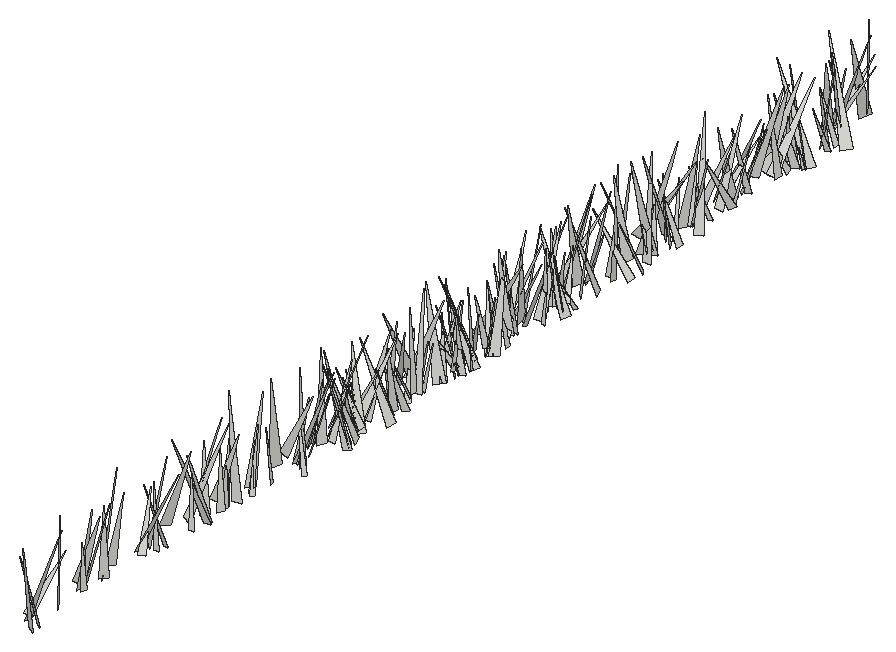
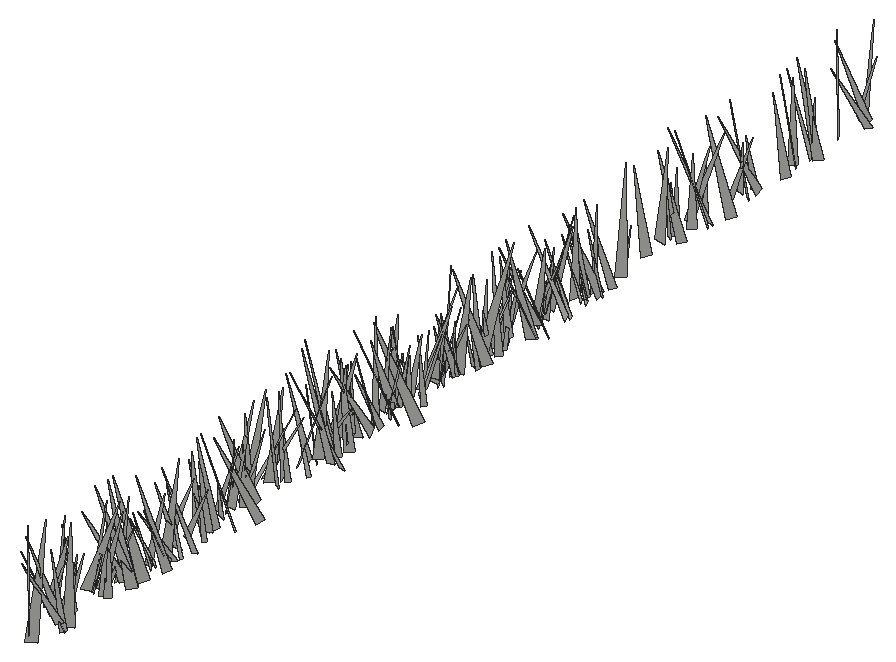
# SketchUp Ruby script. Lengths in inches.
U = 1.inch
M = Sketchup.active_model
def pt(a) = Geom::Point3d.new(a.map { |v| v * U })
def face(e, loops, mat)
  f = e.add_face(loops[0].map { |a| pt(a) })
  loops[1..].each { |l| e.add_face(l.map { |a| pt(a) }).erase! }
  f.material = f.back_material = mat if mat
  f
end
# faces: each face lists its corners as indices into pts; further lists are holes
def faces(e, pts, list, mat = nil) = list.each { |f| face(e, (f[0].is_a?(Array) ? f : [f]).map { |l| l.map { |i| pts[i] } }, mat) }
# xy, xz, yz: faces in a plane at the given z, y or x. An outline is a flat list of corners, or four numbers for a rectangle; further outlines are holes
def ring(l) = l.size == 4 ? [[l[0], l[1]], [l[2], l[1]], [l[2], l[3]], [l[0], l[3]]] : l.each_slice(2).to_a
def flat(e, list, mat, &to3) = list.each { |f| face(e, (f[0].is_a?(Array) ? f : [f]).map { |l| ring(l).map { |u, v| to3.(u, v) } }, mat) }
def xy(e, z, list, mat = nil) = flat(e, list, mat) { |x, y| [x, y, z] }
def xz(e, y, list, mat = nil) = flat(e, list, mat) { |x, z| [x, y, z] }
def yz(e, x, list, mat = nil) = flat(e, list, mat) { |y, z| [x, y, z] }
def lines(e, pts, list) = list.each { |a, b| e.add_line(pt(pts[a]), pt(pts[b])) }
# prism: a flat outline (further loops are holes) pulled along v
def prism(e, loops, v, mat = nil)
  f = face(e, loops, mat); d = Geom::Vector3d.new(v.map { |x| x * U })
  f.pushpull(f.normal.samedirection?(d) ? d.length : -d.length)
end
def box(e, o, s, mat = nil) = prism(e, [[o, [o[0] + s[0], o[1], o[2]], [o[0] + s[0], o[1] + s[1], o[2]], [o[0], o[1] + s[1], o[2]]]], [0, 0, s[2]], mat)
def at(x, y, z, deg = 0) = Geom::Transformation.translation(pt([x, y, z])) * Geom::Transformation.rotation(ORIGIN, Z_AXIS, deg.degrees)
def axes(o, x, y, z) = Geom::Transformation.new([*x, 0, *y, 0, *z, 0, *pt(o).to_a, 1])
def part(name) = M.definitions.add(name)
# library, detail: a bought-in or finely detailed component or shape, given as its bounding box
def library(name, o, s) = part(name).tap { |d| box(d.entities, o, s) }
def detail(e, o, s) = box(e.add_group.entities, o, s)
def put(e, d, t, mat = nil) = e.add_instance(d, t).tap { |i| i.material = mat if mat }
def group(e, t, mat = nil) = e.add_group.tap { |g| g.transformation = t; g.material = mat if mat }.entities
root = M.entities
c1 = part("fur_instance\#9")
p = [[0.8125,0,1.79],[0.67,-0.02,1.48],[0,-0.11,0],[0,0.11,0]]
faces(c1.entities,p,[[0,1,2,3]])
put(root,c1,axes([157.47,112.2,-27.1],[-4.17455,0.44699,1.70239],[0.80041,4.38471,0.81146],[1.56757,-1.04848,4.11925]))
put(root,c1,axes([157.79,64.41,-28.22],[-3.70453,-1.18645,1.17686],[-1.32576,3.8289,-0.31316],[1.01735,0.66938,3.87726]))
put(root,c1,axes([155.74,183.69,-28.22],[3.44417,-6.15496,0.43731],[-6.17002,-3.42915,0.33004],[0.07525,0.54268,7.04535]))
put(root,c1,axes([158.09,92.44,-28.22],[-4.08982,2.78235,0.32679],[2.66533,4.04258,-1.06229],[0.86271,0.7007,4.83111]))
put(root,c1,axes([156.51,123.77,-27.1],[4.13906,-0.88394,1.08396],[-0.87234,-4.27812,-0.15771],[-1.09332,0.06702,4.22946]))
put(root,c1,axes([155.58,185.05,-28.22],[5.53978,-0.90724,0.62547],[-0.85463,-5.56113,-0.49688],[-0.69563,-0.39269,5.59154]))
put(root,c1,axes([157.55,75.13,-27.1],[6.19428,-1.57461,3.33029],[-1.87234,-6.95675,0.19327],[-3.17247,1.03131,6.38836]))
put(root,c1,axes([157.63,117.22,-27.1],[3.93388,5.26717,1.14139],[4.90502,-4.08461,1.94372],[-2.23307,0.30691,6.28017]))
put(root,c1,axes([153.48,151.58,-27.1],[5.8756,3.65861,0.2575],[3.32747,-5.11292,-3.2803],[1.54262,-2.90637,6.0949]))
put(root,c1,axes([159.0625,112.28,-28.22],[-5.62081,-1.07857,0.79033],[-1.22962,5.511,-1.22409],[0.52534,1.35906,5.59093]))
put(root,c1,axes([155.79,118.01,-27.1],[4.34496,-0.35551,0.43941],[-0.4633,-4.19131,1.19014],[-0.32376,1.22666,4.19388]))
put(root,c1,axes([155.21,79.86,-27.1],[6.72288,3.05704,0.61475],[3.02645,-6.7488,0.46346],[-0.75102,0.16938,7.37074]))
put(root,c1,axes([157.85,82.52,-28.22],[-2.17091,-2.72609,1.07786],[-2.90812,2.17161,-0.36485],[0.36901,1.07644,3.46573]))
put(root,c1,axes([157.48,28.99,-27.1],[5.31201,5.41879,2.20999],[5.24419,-5.73235,1.45032],[-2.59727,-0.49162,7.44831]))
put(root,c1,axes([157.34,50.82,-27.1],[2.70237,-4.42657,2.31196],[-4.83243,-2.98105,-0.05917],[-1.25989,1.93941,5.18593]))
put(root,c1,axes([156.33,124.09,-28.22],[3.53738,-5.32848,1.99163],[-5.66565,-3.51029,0.67133],[-0.50966,2.039,6.36044]))
put(root,c1,axes([158.61,155.47,-28.22],[-0.5806,-4.0301,0.94816],[-3.96701,0.26756,-1.29192],[-1.18471,1.07913,3.86131]))
put(root,c1,axes([156.16,32.51,-27.1],[5.31281,-2.73186,1.51927],[-2.91837,-5.40827,0.48055],[-1.11999,1.13346,5.95467]))
put(root,c1,axes([159.02,142.16,-27.1],[-5.68888,-0.08485,0.69236],[-0.12916,5.71868,-0.36046],[0.68548,0.37338,5.67808]))
put(root,c1,axes([158.48,82.14,-28.22],[-4.49758,4.50366,1.60112],[4.72062,4.53017,0.51777],[0.74986,-1.50644,6.34374]))
put(root,c1,axes([158.22,98.96,-28.22],[-5.45216,4.70878,2.71596],[5.23215,5.58914,0.81316],[1.47433,-2.42158,7.15803]))
put(root,c1,axes([158.49,56.12,-27.1],[-0.94907,-6.99906,3.73248],[-7.88487,0.42284,-1.21201],[-0.8643,3.82797,6.95835]))
put(root,c1,axes([153.68,146.02,-28.22],[4.55,-4.60588,0.41001],[-4.16176,-3.82822,3.1795],[2.01545,2.49305,5.6398]))
put(root,c1,axes([157.15,95.66,-27.1],[4.52461,-6.7861,0.00105],[-6.53347,-4.35651,-2.20405],[-1.83437,-1.22185,7.85273]))
put(root,c1,axes([156.55,70.85,-28.22],[2.00613,4.44684,1.43472],[4.67253,-1.91449,-0.59961],[-0.01581,-1.5549,4.84142]))
put(root,c1,axes([154.18,128.22,-28.22],[3.82071,6.83533,0.31448],[6.59967,-3.58608,-2.23672],[1.80694,-1.35528,7.50444]))
put(root,c1,axes([154.97,83.86,-28.22],[3.75203,3.55416,0.24846],[3.4305,-3.50645,-1.64561],[0.96201,-1.35805,4.89916]))
put(root,c1,axes([155.06,129.59,-27.1],[-0.81294,-7.33898,4.00432],[-7.82592,2.08335,2.22952],[2.94113,3.51498,7.03923]))
put(root,c1,axes([158.54,148.17,-28.22],[0.48963,4.22721,0.04806],[3.94805,-0.47454,1.51627],[-1.51146,0.12987,3.97618]))
put(root,c1,axes([159.07,49.21,-27.1],[-1.75901,-6.72397,0.92553],[-6.70142,1.56883,-1.33876],[-1.07676,1.22044,6.82009]))
put(root,c1,axes([156.52,66.78,-27.1],[6.94101,-3.43299,1.84422],[-3.2352,-7.17632,-1.18245],[-2.17258,-0.28153,7.65277]))
put(root,c1,axes([157.6,37.26,-27.1],[-2.09366,4.25191,0.8072],[4.26644,2.17826,-0.40798],[0.72654,-0.53866,4.72184]))
put(root,c1,axes([155.98,161.09,-28.22],[-0.54715,4.89077,0.10405],[4.53126,0.54616,-1.84371],[1.84341,0.10915,4.56287]))
put(root,c1,axes([158.66,108.89,-28.22],[-1.86757,4.60063,0.33127],[4.58089,1.80817,0.71369],[-0.53944,-0.57279,4.91369]))
put(root,c1,axes([158.64,41.03,-27.1],[-2.25031,-4.2676,0.76277],[-4.32128,2.13921,-0.77999],[-0.34742,1.03417,4.76108]))
put(root,c1,axes([158.95,81.81,-27.1],[-4.51725,1.3418,0.80765],[1.52463,4.33149,1.33117],[0.35811,-1.51528,4.52039]))
put(root,c1,axes([158.38,39.37,-27.1],[0.93593,4.40998,1.37185],[4.37962,-1.29175,1.16453],[-1.46587,-1.0437,4.3552]))
put(root,c1,axes([157.36,152.39,-28.22],[-2.00411,5.21831,1.67163],[5.38658,2.20263,-0.41796],[1.00489,-1.39973,5.57427]))
put(root,c1,axes([153.78,112.64,-28.22],[6.07863,-4.42165,0.21276],[-4.21796,-5.67554,2.55792],[1.3435,2.18706,7.06807]))
put(root,c1,axes([156.63,138.79,-27.1],[-3.30417,-4.76212,3.2823],[-5.25525,4.05058,0.5865],[2.41528,2.29867,5.7664]))
put(root,c1,axes([158.08,70.5625,-28.22],[-6.67663,-0.80436,2.4344],[-1.05353,7.05179,-0.55944],[2.33738,0.88086,6.7016]))
put(root,c1,axes([158.02,164.22,-28.22],[0.08099,-5.17118,1.20761],[-5.27072,-0.22549,-0.61212],[-0.64729,1.18913,5.13546]))
put(root,c1,axes([160.05,174.42,-28.22],[-5.06971,5.94983,1.91077],[6.22333,4.58369,2.23904],[-0.56711,-2.88838,7.48926]))
put(root,c1,axes([156.17,154.67,-28.22],[0.84418,-3.62493,0.18375],[-3.45271,-0.74384,1.18829],[1.11924,0.43944,3.52714]))
put(root,c1,axes([155.01,45.44,-27.1],[6.03076,-3.95506,0.64167],[-4.00583,-5.92637,1.12057],[0.08689,1.28836,7.12438]))
put(root,c1,axes([157.19,118.1875,-28.22],[6.83312,3.40706,1.30672],[2.45514,-6.34476,3.70451],[-2.69961,2.8536,6.67654]))
put(root,c1,axes([155.23,157.86,-28.22],[2.52048,5.79703,1.2985],[5.75928,-2.03853,-2.07834],[1.45681,-1.97061,5.96983]))
put(root,c1,axes([155.59,160.3,-28.22],[4.89387,1.35478,0.49174],[1.44124,-4.60961,-1.64362],[-0.00784,-1.71558,4.80457]))
put(root,c1,axes([158.59,92.4,-27.1],[-3.47143,-2.84551,0.09651],[-2.81271,3.45107,0.57956],[0.4415,-0.38766,4.45106]))
put(root,c1,axes([156.99,161.96,-28.22],[3.26606,-6.16963,0.62937],[-6.14796,-3.31446,-0.58694],[-0.81426,0.27855,6.95607]))
put(root,c1,axes([158.59,106.58,-28.22],[-5.73536,-5.62008,0.65862],[-5.46135,5.74328,1.44982],[1.48081,-0.58562,7.89796]))
put(root,c1,axes([158.91,13.99,-27.1],[-3.27995,-3.84872,1.10692],[-4.00472,3.15616,-0.89264],[0.01123,1.42196,4.97734]))
put(root,c1,axes([158.91,183.92,-27.1],[-3.27995,-3.84872,1.10692],[-4.00472,3.15616,-0.89264],[0.01123,1.42196,4.97734]))
put(root,c1,axes([156.54,126.08,-28.22],[4.24921,-1.39082,0.67887],[-1.35455,-4.30166,-0.33452],[-0.74864,-0.11098,4.4585]))
put(root,c1,axes([158.44,93.38,-27.1],[-5.81537,-0.03657,1.70774],[-0.23888,6.01751,-0.6846],[1.69135,0.72416,5.77505]))
put(root,c1,axes([158.31,102.99,-28.22],[-4.48519,-3.52054,0.94744],[-3.42145,4.58335,0.83384],[1.25916,-0.08621,5.64055]))
put(root,c1,axes([156.49,75.13,-27.1],[4.35259,2.65064,0.87547],[2.69973,-4.40951,-0.0717],[-0.70982,-0.51745,5.09567]))
put(root,c1,axes([158.14,54.52,-27.1],[1.43677,3.63281,1.03111],[3.57622,-1.66329,0.8769],[-1.21291,-0.60083,3.80693]))
put(root,c1,axes([157.74,180.98,-28.22],[-1.67476,-3.89018,1.26522],[-4.03938,1.78862,0.15259],[0.64624,1.09838,4.23261]))
put(root,c1,axes([157.96,100.26,-27.1],[1.56672,2.93333,1.48069],[3.11219,-1.85095,0.37383],[-1.05412,-1.105,3.30444]))
put(root,c1,axes([156.88,100.88,-27.1],[4.55494,-1.38322,1.77977],[-1.90749,-4.50337,1.38185],[-1.20098,1.9065,4.55536]))
put(root,c1,axes([158.19,112.65,-27.1],[-3.4412,6.39637,0.09759],[6.32165,3.41718,-1.06042],[0.97968,0.41743,7.18546]))
put(root,c1,axes([158.67,173.29,-28.22],[0.96308,-5.75121,1.64983],[-5.7805,-1.32563,-1.24675],[-1.54408,1.37555,5.69645]))
put(root,c1,axes([156.55,73.67,-27.1],[4.95919,2.18923,1.00137],[2.21006,-5.04934,0.09393],[-0.95452,-0.31696,5.4201]))
put(root,c1,axes([154.92,164.02,-28.22],[6.75875,-1.16964,0.00047],[-1.16859,-6.75255,0.29358],[0.0496,0.28936,6.85293]))
put(root,c1,axes([157.71,158.37,-28.22],[0.77683,6.56918,0.32302],[6.56801,-0.79193,0.30978],[-0.34589,-0.28401,6.60769]))
put(root,c1,axes([156.57,84.83,-28.22],[3.10305,4.72146,0.30771],[4.72969,-3.10544,-0.04628],[-0.13026,-0.28259,5.64969]))
put(root,c1,axes([157.29,164.5625,-28.22],[3.89268,2.82638,0.90518],[2.67493,-3.98806,0.94914],[-1.28551,0.26015,4.71599]))
put(root,c1,axes([158.48,102.09,-27.1],[2.70067,-3.13661,0.88183],[-2.51329,-2.73437,-2.02883],[-2.07348,-0.77102,3.60774]))
put(root,c1,axes([156.36,48.83,-27.1],[5.62974,5.25868,1.12192],[5.27805,-5.71471,0.30107],[-1.02693,-0.54292,7.69786]))
put(root,c1,axes([158.54,99.46,-28.22],[-4.5869,1.43943,1.05541],[1.33614,4.69877,-0.60151],[1.18347,0.27406,4.76967]))
put(root,c1,axes([157.04,81.8125,-27.1],[-0.66532,-4.77379,0.4836],[-4.67341,0.75535,1.0268],[1.0873,0.32553,4.70929]))
put(root,c1,axes([160.52,138.84,-28.22],[-5.4011,-4.4458,0.12135],[-4.40164,5.31613,-1.14717],[-0.63674,0.96192,6.9008]))
put(root,c1,axes([158.79,134.85,-28.22],[-7.37531,-1.40171,2.74866],[-2.16749,7.42249,-2.03071],[2.19589,2.61858,7.22747]))
put(root,c1,axes([159.3125,131.0625,-28.22],[-6.20771,-3.16783,0.82777],[-3.08728,6.25411,0.78157],[1.09042,-0.32718,6.92531]))
put(root,c1,axes([156.02,15.29,-27.1],[-0.77489,5.32124,0.74593],[4.8544,1.01638,-2.20776],[2.30365,-0.35187,4.90325]))
put(root,c1,axes([156.02,185.21,-27.1],[-0.77489,5.32124,0.74593],[4.8544,1.01638,-2.20776],[2.30365,-0.35187,4.90325]))
put(root,c1,axes([156.64,174.39,-28.22],[3.91329,-2.80057,0.16354],[-2.76188,-3.89534,-0.61821],[-0.49189,-0.40864,4.7723]))
put(root,c1,axes([156.87,25.13,-27.1],[6.13024,0.22864,1.74835],[0.20896,-6.37456,0.10097],[-1.75081,0.03976,6.13367]))
put(root,c1,axes([157.33,60.35,-27.1],[-5.57842,3.33095,2.99608],[3.28064,6.29556,-0.89096],[3.05108,-0.67911,6.43585]))
put(root,c1,axes([157.11,129.6,-27.1],[6.05759,-4.04132,1.47541],[-3.82561,-6.22554,-1.34569],[-1.96821,-0.33746,7.15653]))
put(root,c1,axes([158.96,80.94,-28.22],[2.56501,3.25674,2.5986],[3.3721,-3.41499,0.95138],[-2.44704,-1.29222,4.03491]))
put(root,c1,axes([159.47,104.85,-28.22],[-5.95975,2.47486,1.75961],[2.91321,5.75356,1.77469],[0.85695,-2.34763,6.20435]))
put(root,c1,axes([156.4375,74.08,-27.1],[5.73568,-0.06882,1.05766],[0.01363,-5.81521,-0.45231],[-1.05981,-0.44725,5.71823]))
put(root,c1,axes([157.63,25.0625,-27.1],[3.35457,-1.66316,1.27005],[-1.64462,-3.57909,-0.343],[-1.29397,0.23728,3.72849]))
put(root,c1,axes([157.97,53.91,-27.1],[-2.87037,3.7349,1.34525],[3.80013,3.06525,-0.40189],[1.14815,-0.80807,4.69329]))
put(root,c1,axes([157.9,144.2,-28.22],[-2.69115,3.5868,1.84623],[3.86426,2.92918,-0.05799],[1.15809,-1.43902,4.48375]))
put(root,c1,axes([157.51,174.43,-28.22],[1.04102,-4.92803,1.21287],[-5.07408,-1.03535,0.14838],[-0.10125,1.21771,5.0346]))
put(root,c1,axes([158.19,138.52,-27.1],[-6.01027,1.97565,2.91231],[2.62602,6.35479,1.10849],[2.3428,-2.05464,6.22879]))
put(root,c1,axes([159.04,181.29,-28.22],[-4.29082,0.07848,0.62907],[0.12494,4.3243,0.31276],[0.62151,-0.32753,4.28013]))
put(root,c1,axes([156.87,96.3,-28.22],[4.1341,0.32333,0.78637],[0.3951,-4.18703,-0.35553],[-0.75288,-0.42186,4.13146]))
put(root,c1,axes([156.06,77.87,-28.22],[4.46845,1.48023,0.19389],[1.49287,-4.43008,-0.58427],[0.00126,-0.6156,4.67084]))
put(root,c1,axes([157.32,163.58,-28.22],[3.29969,3.36632,0.10349],[3.25213,-3.22241,1.12716],[-0.87548,0.71745,4.57707]))
put(root,c1,axes([158.87,93.67,-27.1],[0.5538,7.06628,1.29605],[7.05626,-0.7792,1.23321],[-1.34954,-1.17443,6.97985]))
put(root,c1,axes([156.96,151.4375,-28.22],[6.61649,-1.70465,2.3436],[-2.13195,-6.81989,1.0584],[-1.96294,1.66119,6.75008]))
put(root,c1,axes([158.46,123.48,-27.1],[-4.8782,2.33838,1.88669],[2.5546,5.12175,0.25721],[1.58166,-1.06025,5.40358]))
put(root,c1,axes([157.9,147.11,-27.1],[-0.40558,-7.48594,0.6627],[-7.51279,0.42075,0.15485],[0.19107,0.65318,7.49532]))
put(root,c1,axes([155.63,168.05,-28.22],[6.10397,-4.61293,1.81963],[-4.95361,-5.80478,1.9013],[-0.22786,2.62185,7.41098]))
put(root,c1,axes([159.83,77.6875,-28.22],[-0.65544,-6.57541,2.82853],[-6.91722,-0.14862,-1.94837],[-1.84083,2.89967,6.31422]))
put(root,c1,axes([158.56,172.01,-28.22],[-4.22388,-0.55824,1.0602],[-0.01996,3.91714,1.98304],[1.19803,-1.90295,3.77099]))
put(root,c1,axes([160.77,181.35,-28.22],[-3.56857,7.17935,0.49748],[7.02506,3.35468,1.97986],[-1.56176,-1.31463,7.76903]))
put(root,c1,axes([158.45,169.9,-28.22],[5.59524,-0.57904,3.08549],[-0.36766,-6.38318,-0.53118],[-3.11775,-0.28642,5.59999]))
put(root,c1,axes([159.71,125.71,-28.22],[-0.53868,-3.7535,0.51973],[-3.36849,0.23389,-1.80211],[-1.73555,0.71104,3.33637]))
put(root,c1,axes([155.44,96.09,-27.1],[4.70932,-5.02611,1.74089],[-5.27526,-4.11549,2.38842],[0.68127,2.87596,6.46026]))
put(root,c1,axes([157.375,90.03,-28.22],[4.05773,-0.76512,0.97615],[-0.40955,-3.97873,-1.41614],[-1.1707,-1.26007,3.87881]))
put(root,c1,axes([156.31,108.39,-28.22],[4.66467,-0.77947,0.02704],[-0.7406,-4.47818,-1.32848],[-0.24456,-1.30606,4.53893]))
put(root,c1,axes([157.875,111.09,-27.1],[3.73887,4.62596,1.90486],[4.75099,-4.02818,0.45718],[-1.5672,-1.17533,5.9304]))
put(root,c1,axes([155.71,170.51,-28.22],[4.37755,-6.1842,1.75356],[-6.40379,-4.01166,1.83857],[0.55746,2.47882,7.3503]))
put(root,c1,axes([156.91,101.11,-27.1],[-0.57371,3.97778,1.97621],[4.19128,1.14438,-1.08668],[1.47014,-1.71025,3.86924]))
put(root,c1,axes([157.14,142.68,-28.22],[7.73551,0.03019,2.73159],[-1.01366,-7.58581,2.95441],[-2.53672,3.12332,7.14916]))
put(root,c1,axes([158.25,108.75,-27.1],[1.30026,-4.12004,1.09762],[-4.18224,-1.45572,-0.50983],[-0.82967,0.8811,4.29016]))
put(root,c1,axes([156.68,39.93,-27.1],[-3.91032,-4.73518,3.93684],[-5.20514,5.03349,0.88414],[3.29046,2.33522,6.07707]))
put(root,c1,axes([159.94,151.28,-28.22],[0.30584,8.28043,0.48557],[7.987,-0.4251,2.21855],[-2.2381,-0.38549,7.98355]))
put(root,c1,axes([156.11,169.82,-28.22],[-0.17327,7.80384,1.95788],[7.72096,0.71202,-2.15474],[2.26272,-1.83203,7.50246]))
put(root,c1,axes([159.12,102.66,-28.22],[0.3865,-5.10308,2.42648],[-5.49086,-0.91339,-1.04632],[-1.33405,2.28099,5.00959]))
put(root,c1,axes([159.33,104.625,-28.22],[-5.30333,-1.20318,1.41609],[-1.56427,5.2022,-1.4382],[1.00301,1.75149,5.24448]))
put(root,c1,axes([160.55,136.46,-28.22],[-5.67147,0.82087,0.04901],[0.80443,5.46726,1.5178],[-0.17066,-1.50898,5.5259]))
put(root,c1,axes([156.76,73.66,-28.22],[4.65489,2.00226,0.76997],[2.06003,-4.68544,-0.26978],[-0.59848,-0.55448,5.06006]))
put(root,c1,axes([157.6875,88.79,-27.1],[5.90361,-0.69248,2.28384],[-0.937,-6.27702,0.51884],[-2.19488,0.81708,5.9214]))
put(root,c1,axes([158.9,49.66,-27.1],[-0.82643,-5.48525,0.94931],[-5.54864,0.73423,-0.58792],[-0.44918,1.02229,5.51591]))
put(root,c1,axes([155.74,93.35,-27.1],[6.93671,-0.62868,0.23505],[-0.51232,-6.5363,-2.3628],[-0.4336,-2.33453,6.55213]))
put(root,c1,axes([159.5,174.07,-28.22],[-4.59653,-5.39297,2.39685],[-5.86856,4.49796,-1.13384],[0.62378,2.57709,6.99476]))
put(root,c1,axes([158.375,143.41,-28.22],[1.61042,-7.88282,1.5376],[-7.97737,-1.75156,-0.62458],[-0.92985,1.37466,8.02136]))
put(root,c1,axes([158.36,113.35,-27.1],[-2.64442,5.36733,3.49605],[6.32318,2.79183,0.49668],[1.02376,-3.3795,5.96276]))
put(root,c1,axes([155.4,69.84,-27.1],[1.83372,-5.8574,1.52699],[-5.60076,-1.03656,2.74963],[2.29617,2.14936,5.48737]))
put(root,c1,axes([158.94,119.91,-28.22],[1.77865,4.09096,1.0407],[3.89915,-2.02489,1.29578],[-1.61729,-0.38272,4.26855]))
put(root,c1,axes([158.72,101.15,-27.1],[-4.5247,0.14497,1.56827],[-0.47946,4.4174,-1.79167],[1.5002,1.84904,4.15738]))
put(root,c1,axes([156.78,14.41,-27.1],[6.71372,1.26121,1.18447],[0.98901,-6.69183,1.51954],[-1.41968,1.3025,6.66001]))
put(root,c1,axes([156.78,184.34,-27.1],[6.71372,1.26121,1.18447],[0.98901,-6.69183,1.51954],[-1.41968,1.3025,6.66001]))
put(root,c1,axes([159.57,173.79,-28.22],[-3.7674,-0.4134,0.34529],[-0.49063,3.64055,-0.99453],[0.22227,1.02903,3.6572]))
put(root,c1,axes([157.58,29.26,-27.1],[-3.8078,3.44308,3.43375],[4.19662,4.52997,0.11149],[2.45637,-2.40193,5.13242]))
put(root,c1,axes([159.28,141.24,-28.22],[1.24745,7.40868,1.63783],[7.39275,-1.56046,1.42803],[-1.70827,-1.34297,7.376]))
put(root,c1,axes([157.89,96.03,-28.22],[1.71748,3.11444,0.84575],[3.20742,-1.75327,-0.057],[-0.35706,-0.7688,3.55615]))
put(root,c1,axes([156.57,85.46,-28.22],[3.44666,-5.98968,2.82803],[-6.61551,-2.95389,1.80641],[0.33028,3.33943,6.67028]))
put(root,c1,axes([157.71,113.75,-28.22],[-1.72893,-3.46771,1.76985],[-3.62718,2.13831,0.64633],[1.41454,1.24466,3.82053]))
put(root,c1,axes([158.9,159.82,-28.22],[2.87484,-4.36178,0.57915],[-3.91954,-2.85297,-2.03053],[-1.99945,-0.67874,4.81319]))
put(root,c1,axes([158.51,146.05,-27.1],[-3.07714,-3.38347,1.94932],[-3.73457,3.27489,-0.21099],[1.14047,1.59489,4.5686]))
put(root,c1,axes([157.63,135.36,-28.22],[0.94774,-3.5048,1.15841],[-3.67796,-0.79512,0.60341],[0.31324,1.26803,3.58018]))
put(root,c1,axes([159.375,80.19,-28.22],[-5.8236,-1.97497,1.08531],[-1.72724,5.8434,1.36532],[1.44743,-0.9731,5.99589]))
put(root,c1,axes([157.15,189.85,-28.22],[6.81384,-4.6319,0.82302],[-4.34734,-6.75311,-2.01405],[-1.7979,-1.22528,7.98915]))
put(root,c1,axes([156.03,54.54,-27.1],[3.29636,-5.4576,1.30622],[-5.51274,-2.86598,1.93739],[1.04942,2.08768,6.07437]))
put(root,c1,axes([156.74,70.84,-28.22],[6.92746,0.46404,1.30725],[0.06508,-6.75935,2.05449],[-1.38564,2.00246,6.63205]))
put(root,c1,axes([157.5,19.875,-27.1],[6.08028,3.66314,2.96745],[4.34842,-6.22849,-1.22118],[-1.82087,-2.64225,6.99265]))
put(root,c1,axes([157.5,189.81,-27.1],[6.08028,3.66314,2.96745],[4.34842,-6.22849,-1.22118],[-1.82087,-2.64225,6.99265]))
put(root,c1,axes([158.2,76.42,-27.1],[1.54833,5.59255,0.52827],[5.59137,-1.58705,0.41342],[-0.54067,-0.39706,5.78818]))
put(root,c1,axes([158.46,160.5,-28.22],[2.63197,4.07891,0.20518],[3.86496,-2.5665,1.44292],[-1.31973,0.61842,4.63495]))
put(root,c1,axes([158.1875,108.875,-28.22],[3.3556,2.16226,1.21696],[2.08771,-3.56664,0.58052],[-1.34083,-0.14202,3.94948]))
put(root,c1,axes([158.39,52.87,-27.1],[-3.98978,2.11987,2.03955],[2.3526,4.36264,0.06771],[1.76604,-1.02247,4.51748]))
put(root,c1,axes([156.22,114.16,-28.22],[4.64022,6.0526,0.40907],[6.0581,-4.59639,-0.71102],[0.31728,-0.75645,7.59342]))
put(root,c1,axes([160.21,86.36,-28.22],[-6.51837,1.52305,1.37348],[1.82295,6.39951,1.5551],[0.93967,-1.84981,6.5108]))
put(root,c1,axes([157.97,121.47,-27.1],[0.13174,-4.85064,1.64659],[-5.10405,0.01535,0.4536],[0.43432,1.65178,4.83118]))
put(root,c1,axes([159.04,58.67,-27.1],[-3.45785,1.40655,0.59459],[1.25916,3.45892,-0.85969],[0.86397,0.58836,3.63264]))
put(root,c1,axes([158.06,128.78,-28.22],[3.88828,4.27161,1.82836],[4.44707,-4.1121,0.14976],[-1.3465,-1.2459,5.77433]))
put(root,c1,axes([155.875,26.125,-27.1],[2.64878,-6.42579,1.07864],[-6.29914,-2.22772,2.19734],[1.66585,1.79353,6.59382]))
put(root,c1,axes([156.875,26.32,-27.1],[6.30339,2.19635,1.13005],[2.22882,-6.39265,-0.00763],[-1.06457,-0.37914,6.67507]))
put(root,c1,axes([156.08,127.84,-27.1],[7.78659,2.72532,1.24866],[2.87625,-7.77148,-0.97412],[-0.84485,-1.33952,8.19204]))
put(root,c1,axes([158.98,146.59,-28.22],[-3.81411,-2.18756,1.38745],[-2.30966,3.98998,-0.05835],[1.17299,0.74331,4.39652]))
put(root,c1,axes([156.39,48.22,-27.1],[3.64323,6.95762,0.66244],[6.95502,-3.53547,-1.11744],[0.68929,-1.10109,7.77386]))
put(root,c1,axes([158.66,46.38,-27.1],[-0.06677,3.94377,1.582],[4.24655,0.00562,0.16522],[-0.15123,-1.5834,3.94087]))
put(root,c1,axes([156.25,132.58,-28.22],[5.4983,0.81734,0.21266],[0.84397,-5.26527,-1.58403],[0.03145,-1.59793,5.32824]))
put(root,c1,axes([157.91,120.34,-28.22],[-1.91497,6.86191,1.78883],[6.91485,2.21764,-1.10438],[1.57179,-1.39609,7.03799]))
put(root,c1,axes([159.18,109.38,-28.22],[-5.92088,3.75972,1.43779],[3.50525,6.07307,-1.44586],[1.97886,0.49178,6.86307]))
put(root,c1,axes([160.08,123.2,-28.22],[-6.07802,2.92755,1.98205],[3.37511,5.97833,1.51972],[1.05246,-2.26504,6.57292]))
put(root,c1,axes([158.625,114.35,-27.1],[-1.20745,-5.31811,1.49773],[-5.50418,1.29079,0.14593],[0.47907,1.42653,5.45151]))
put(root,c1,axes([158.65,58.95,-27.1],[0.70725,4.81258,1.31899],[4.97344,-0.78845,0.21001],[-0.40688,-1.27212,4.85974]))
put(root,c1,axes([158.15,124.95,-28.22],[-3.5454,-4.09399,1.47684],[-3.82101,3.83994,1.47185],[2.08366,0.07566,5.21193]))
put(root,c1,axes([155.5,185.05,-28.22],[3.84668,4.92623,0.09388],[4.62666,-3.57049,-2.21792],[1.69428,-1.43435,5.84342]))
put(root,c1,axes([156.54,37.73,-27.1],[6.37696,0.70596,0.43543],[0.57496,-6.19552,1.62437],[-0.59783,1.57187,6.20688]))
put(root,c1,axes([157.58,169.64,-28.22],[-2.00066,7.03095,0.19663],[6.73059,1.97306,-2.06922],[2.04255,0.38513,7.01108]))
put(root,c1,axes([159.67,68.77,-28.22],[-0.43735,3.78387,0.74816],[3.7266,0.2203,1.06426],[-0.99494,-0.83814,3.65736]))
put(root,c1,axes([157.5,131.0625,-27.1],[6.67173,1.075,1.66778],[0.88806,-6.84957,0.86244],[-1.77439,0.61387,6.70252]))
put(root,c1,axes([158.1,102.1875,-28.22],[-5.2101,-5.93708,2.74108],[-5.84341,5.80017,1.45611],[2.93548,1.00834,7.76362]))
put(root,c1,axes([158.93,124.81,-27.1],[-1.59242,3.59476,0.56652],[3.61736,1.63113,-0.18207],[0.39739,-0.44291,3.92746]))
put(root,c1,axes([158.23,88.91,-28.22],[-1.70648,-4.83175,0.15849],[-4.67215,1.69151,1.26205],[1.24174,-0.27565,4.96639]))
put(root,c1,axes([158.19,89.35,-28.22],[5.03393,-2.19184,1.50174],[-1.99616,-5.24318,-0.96135],[-1.75349,-0.32355,5.40559]))
put(root,c1,axes([159.95,147.33,-28.22],[-5.1344,0.67452,1.09766],[0.89094,5.11676,1.02317],[0.93062,-1.17714,5.07643]))
put(root,c1,axes([158.16,53.88,-27.1],[2.54214,-2.62214,0.84113],[-2.70032,-2.59808,0.06187],[-0.53981,0.64801,3.65161]))
put(root,c1,axes([157.55,180.11,-28.22],[5.68987,2.39384,1.65752],[2.61602,-5.80047,-0.60296],[-1.2784,-1.21517,6.14342]))
put(root,c1,axes([156.99,83.58,-27.1],[0.07577,6.70614,0.84141],[6.48392,0.16538,-1.90197],[1.90764,-0.82847,6.43122]))
put(root,c1,axes([159.55,78.67,-28.22],[-5.81163,-3.8947,1.27527],[-3.71182,5.94036,1.22659],[1.73708,-0.33677,6.88761]))
put(root,c1,axes([158.16,123.76,-27.1],[-3.52584,-3.38703,1.52089],[-2.9555,3.82986,1.67745],[2.24724,-0.27722,4.59235]))
put(root,c1,axes([157.64,153.08,-28.22],[5.31059,0.52385,1.16283],[0.52648,-5.43598,0.04446],[-1.16164,-0.06886,5.33618]))
put(root,c1,axes([159.28,90.6,-28.22],[1.87791,-4.76016,0.94457],[-4.63856,-2.05833,-1.15104],[-1.42657,0.4266,4.98606]))
put(root,c1,axes([157.37,117.34,-27.1],[7.02659,-0.33713,1.59],[0.09653,-6.95626,-1.90152],[-1.62247,-1.87389,6.7728]))
put(root,c1,axes([158.52,103.31,-27.1],[1.07632,-4.38935,0.89904],[-4.4763,-1.09335,0.02097],[-0.19334,0.87825,4.51934]))
put(root,c1,axes([159.03,179.52,-28.22],[0.58704,-3.79537,0.45103],[-3.78334,-0.64184,-0.47675],[-0.5428,0.36891,3.81079]))
put(root,c1,axes([158.65,12.55,-27.1],[-3.10043,-5.65859,2.0595],[-5.81568,3.41455,0.62657],[1.56175,1.48157,6.42182]))
put(root,c1,axes([158.65,182.48,-27.1],[-3.10043,-5.65859,2.0595],[-5.81568,3.41455,0.62657],[1.56175,1.48157,6.42182]))
